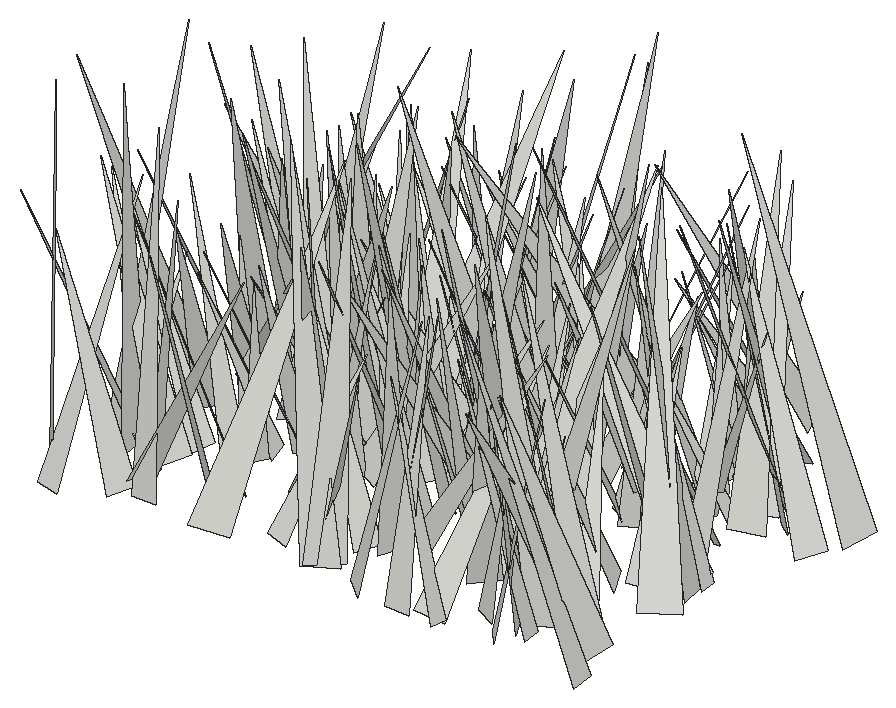
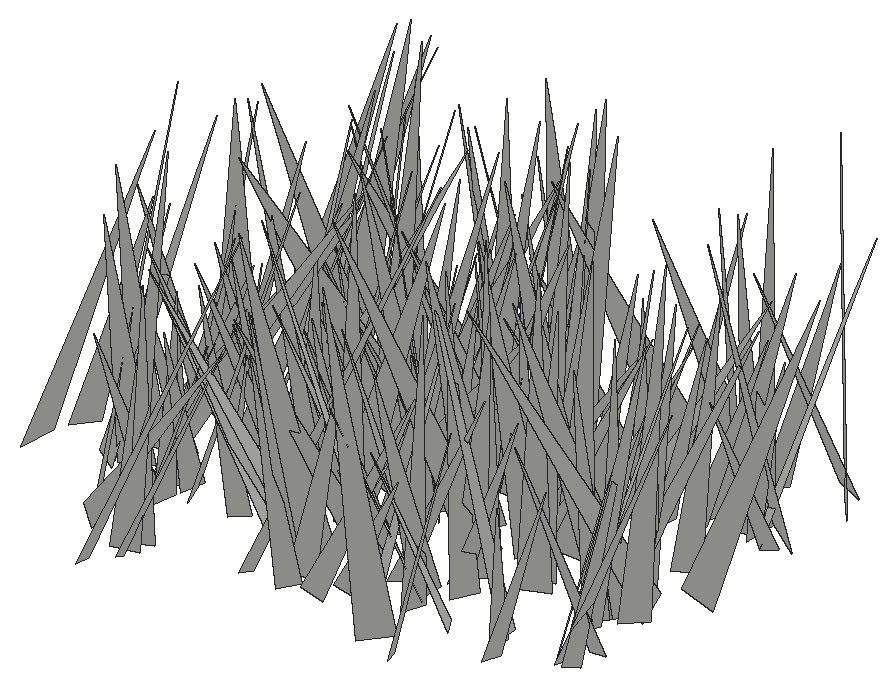
# SketchUp Ruby script. Lengths in inches.
U = 1.inch
M = Sketchup.active_model
def pt(a) = Geom::Point3d.new(a.map { |v| v * U })
def face(e, loops, mat)
  f = e.add_face(loops[0].map { |a| pt(a) })
  loops[1..].each { |l| e.add_face(l.map { |a| pt(a) }).erase! }
  f.material = f.back_material = mat if mat
  f
end
# faces: each face lists its corners as indices into pts; further lists are holes
def faces(e, pts, list, mat = nil) = list.each { |f| face(e, (f[0].is_a?(Array) ? f : [f]).map { |l| l.map { |i| pts[i] } }, mat) }
# xy, xz, yz: faces in a plane at the given z, y or x. An outline is a flat list of corners, or four numbers for a rectangle; further outlines are holes
def ring(l) = l.size == 4 ? [[l[0], l[1]], [l[2], l[1]], [l[2], l[3]], [l[0], l[3]]] : l.each_slice(2).to_a
def flat(e, list, mat, &to3) = list.each { |f| face(e, (f[0].is_a?(Array) ? f : [f]).map { |l| ring(l).map { |u, v| to3.(u, v) } }, mat) }
def xy(e, z, list, mat = nil) = flat(e, list, mat) { |x, y| [x, y, z] }
def xz(e, y, list, mat = nil) = flat(e, list, mat) { |x, z| [x, y, z] }
def yz(e, x, list, mat = nil) = flat(e, list, mat) { |y, z| [x, y, z] }
def lines(e, pts, list) = list.each { |a, b| e.add_line(pt(pts[a]), pt(pts[b])) }
# prism: a flat outline (further loops are holes) pulled along v
def prism(e, loops, v, mat = nil)
  f = face(e, loops, mat); d = Geom::Vector3d.new(v.map { |x| x * U })
  f.pushpull(f.normal.samedirection?(d) ? d.length : -d.length)
end
def box(e, o, s, mat = nil) = prism(e, [[o, [o[0] + s[0], o[1], o[2]], [o[0] + s[0], o[1] + s[1], o[2]], [o[0], o[1] + s[1], o[2]]]], [0, 0, s[2]], mat)
def at(x, y, z, deg = 0) = Geom::Transformation.translation(pt([x, y, z])) * Geom::Transformation.rotation(ORIGIN, Z_AXIS, deg.degrees)
def axes(o, x, y, z) = Geom::Transformation.new([*x, 0, *y, 0, *z, 0, *pt(o).to_a, 1])
def part(name) = M.definitions.add(name)
# library, detail: a bought-in or finely detailed component or shape, given as its bounding box
def library(name, o, s) = part(name).tap { |d| box(d.entities, o, s) }
def detail(e, o, s) = box(e.add_group.entities, o, s)
def put(e, d, t, mat = nil) = e.add_instance(d, t).tap { |i| i.material = mat if mat }
def group(e, t, mat = nil) = e.add_group.tap { |g| g.transformation = t; g.material = mat if mat }.entities
root = M.entities
c1 = part("fur_instance\#9")
p = [[0.8125,0,1.79],[0.67,-0.02,1.48],[0,-0.11,0],[0,0.11,0]]
faces(c1.entities,p,[[0,1,2,3]])
put(root,c1,axes([89.13,415.83,-27.1],[5.01755,-2.86523,2.69296],[-2.1597,-5.65647,-1.99435],[-3.28592,-0.6574,5.42291]))
put(root,c1,axes([90.02,413.82,-27.1],[-7.1325,-1.97369,0.04131],[-1.9512,7.0246,-1.27181],[-0.29997,1.23662,7.29044]))
put(root,c1,axes([67.68,414.45,-27.1],[-4.78062,2.36193,1.12593],[2.54726,4.73726,0.87783],[0.59826,-1.2963,5.25951]))
put(root,c1,axes([64.64,414.03,-27.1],[-5.7343,-4.84539,3.53032],[-5.45543,6.24306,-0.29262],[2.4858,2.5238,7.50162]))
put(root,c1,axes([71.45,415.38,-27.1],[-3.14093,-4.54056,1.19879],[-4.68857,3.11384,-0.49041],[0.26658,1.26749,5.49924]))
put(root,c1,axes([83.08,413.99,-27.1],[-4.76571,-0.2474,0.30777],[-0.30187,4.68534,-0.90794],[0.25457,0.92426,4.68496]))
put(root,c1,axes([86.31,418.15,-27.1],[4.64507,-4.79979,0.2726],[-4.36308,-4.36804,-2.56373],[-2.01887,-1.6035,6.16782]))
put(root,c1,axes([76.08,415.99,-27.1],[5.21952,0.68023,0.61562],[0.83808,-4.98198,-1.60081],[-0.37326,-1.674,5.01433]))
put(root,c1,axes([79.03,414.06,-27.1],[3.65147,4.43575,1.22236],[4.5601,-3.69672,-0.20725],[-0.61278,-1.07778,5.74161]))
put(root,c1,axes([81.28,413.75,-27.1],[0.82489,5.68831,1.342],[5.81529,-0.93413,0.38496],[-0.58339,-1.2684,5.73491]))
put(root,c1,axes([85.58,415.59,-27.1],[3.95748,1.9361,2.48086],[2.44941,-4.39763,-0.47534],[-1.97573,-1.57388,4.37997]))
put(root,c1,axes([84.11,415.45,-27.1],[-0.58036,-3.55618,1.37675],[-3.59236,0.97706,1.00942],[1.27936,1.13031,3.45894]))
put(root,c1,axes([85.32,414.44,-27.1],[3.56693,3.32971,1.1246],[3.34181,-3.70943,0.38354],[-1.08812,-0.47732,4.86445]))
put(root,c1,axes([67.83,415.27,-27.1],[5.28703,-2.12696,0.17156],[-2.11759,-5.17319,1.12251],[0.26309,1.10465,5.58719]))
put(root,c1,axes([79.96,415.2,-27.1],[5.42096,2.25752,1.64956],[2.38588,-5.61122,-0.16143],[-1.45775,-0.7887,5.87002]))
put(root,c1,axes([65.36,412.92,-27.1],[2.05142,5.93925,0.09208],[5.90467,-2.04959,0.65232],[-0.64654,0.12643,6.2496]))
put(root,c1,axes([86.4,415.33,-27.1],[-5.31837,-1.43549,0.4315],[-1.49067,5.23198,-0.96754],[0.15722,1.04767,5.42306]))
put(root,c1,axes([65.6,418.01,-27.1],[-4.61159,-4.4726,0.38091],[-4.39573,4.61032,0.9157],[0.90928,-0.396,6.35865]))
put(root,c1,axes([77.02,414.81,-27.1],[-5.99811,4.4385,2.51735],[4.45899,6.44808,-0.74453],[2.48087,-0.8583,7.4245]))
put(root,c1,axes([77.01,414.55,-27.1],[-1.50956,7.97784,1.83345],[8.07703,1.14872,1.65178],[-1.3301,-2.07864,7.94961]))
put(root,c1,axes([82.47,417.49,-27.1],[4.37125,-4.19897,0.80164],[-4.19734,-4.43318,-0.33332],[-0.81017,0.31203,6.05212]))
put(root,c1,axes([78.4,417.3,-27.1],[5.51508,-3.1001,1.56666],[-3.03836,-5.73026,-0.64316],[-1.68328,0.18611,6.29389]))
put(root,c1,axes([68.75,414.43,-27.1],[1.63726,6.8228,1.57078],[6.72877,-1.9791,1.58281],[-1.9343,-1.10957,6.83563]))
put(root,c1,axes([74.47,415.16,-27.1],[0.4921,4.23207,0.57816],[4.10963,-0.31046,-1.22532],[1.16432,-0.69285,4.08059]))
put(root,c1,axes([82.51,414.16,-27.1],[-2.22642,5.28944,0.76409],[4.89566,2.35054,-2.00661],[2.14349,0.12554,5.37668]))
put(root,c1,axes([67.1,417.14,-27.1],[3.49606,4.56093,2.47636],[5.16488,-3.35013,-1.12142],[-0.50841,-2.67048,5.63622]))
put(root,c1,axes([86.95,417.37,-27.1],[-5.18557,-4.32883,1.54546],[-4.49087,5.26797,-0.31293],[0.97941,1.23577,6.74766]))
put(root,c1,axes([86.36,416.29,-27.1],[-0.9931,7.68396,2.84346],[8.04191,0.36629,1.81887],[-1.56723,-2.98953,7.53135]))
put(root,c1,axes([77.51,416.75,-27.1],[-4.02277,2.62654,1.01722],[2.78428,3.97624,0.74391],[0.42575,-1.18612,4.74637]))
put(root,c1,axes([65.93,417.47,-27.1],[7.3985,0.06507,3.2704],[0.28828,-8.06925,-0.49163],[-3.25831,-0.56619,7.38244]))
put(root,c1,axes([72.08,414.11,-27.1],[-4.61251,5.93847,1.25396],[5.3205,4.71401,-2.75381],[2.92064,0.79104,6.99694]))
put(root,c1,axes([72.86,420.16,-27.1],[5.93446,-4.51627,0.11992],[-4.41947,-5.84426,-1.3935],[-0.93776,-1.03771,7.32616]))
put(root,c1,axes([71.45,417.04,-27.1],[-4.82792,-3.85999,0.34861],[-3.62589,4.30173,-2.58417],[-1.36894,2.21934,5.6152]))
put(root,c1,axes([67.8,417.46,-27.1],[-5.5849,2.54638,0.93821],[2.66389,5.55377,0.78405],[0.51763,-1.10771,6.08773]))
put(root,c1,axes([78.87,418.1875,-27.1],[4.45492,4.83666,0.95124],[4.56601,-3.56591,-3.25273],[1.85733,-2.83468,5.71483]))
put(root,c1,axes([87.88,416.87,-27.1],[-6.93734,1.12272,0.61983],[1.08478,6.95591,-0.45824],[0.68406,0.3553,7.01265]))
put(root,c1,axes([84.2,417.5625,-27.1],[-6.46812,-3.13785,1.21731],[-3.3431,6.29489,-1.53709],[0.38946,1.92167,7.02282]))
put(root,c1,axes([76.34,421.15,-27.1],[-2.99336,-6.46525,0.18966],[-6.30073,2.9619,1.52434],[1.46161,-0.47255,6.9596]))
put(root,c1,axes([74.34,418.125,-27.1],[-5.53367,-3.1899,2.46645],[-3.58117,5.81278,-0.51687],[1.85312,1.70777,6.3663]))
put(root,c1,axes([80.82,418.96,-27.1],[-3.26871,-2.2439,0.63682],[-2.29753,3.28654,-0.21245],[0.40248,0.53729,3.95909]))
put(root,c1,axes([74.2,418.54,-27.1],[-1.49797,-4.88201,2.75569],[-5.27998,2.18724,1.00478],[1.88406,2.24805,5.00683]))
put(root,c1,axes([70.18,419.33,-27.1],[3.44775,-2.42349,1.09947],[-2.43313,-3.5995,-0.30427],[-1.07797,0.37336,4.2033]))
put(root,c1,axes([80.49,419.33,-27.1],[-1.33118,-5.02308,1.66852],[-5.29255,1.28443,-0.35575],[0.06525,1.70478,5.18429]))
put(root,c1,axes([80.43,421.6,-27.1],[7.22069,-3.00234,1.05262],[-2.62839,-7.10035,-2.22196],[-1.79266,-1.6827,7.49769]))
put(root,c1,axes([86.3,420.58,-27.1],[-5.06216,-2.56794,0.53616],[-2.44101,5.03776,1.08155],[0.96086,-0.73072,5.57226]))
put(root,c1,axes([83.34,419.48,-27.1],[3.34183,1.38887,0.77255],[1.56239,-3.2005,-1.00466],[-0.29109,-1.23347,3.4767]))
put(root,c1,axes([67.99,418.83,-27.1],[-4.93751,1.50851,0.32737],[1.53378,4.91815,0.47027],[0.1741,-0.54591,5.14135]))
put(root,c1,axes([66.37,417.86,-27.1],[-3.43494,4.07646,0.13435],[4.04677,3.38429,0.77755],[-0.50915,-0.60283,5.27368]))
put(root,c1,axes([70.38,420.34,-27.1],[-4.26767,-0.91045,0.71231],[-0.70932,4.21373,1.13607],[0.91278,-0.98229,4.21323]))
put(root,c1,axes([79.55,421.67,-27.1],[1.60402,-6.13136,0.73735],[-5.58582,-1.76536,-2.52831],[-2.63361,0.00991,5.81155]))
put(root,c1,axes([78.98,418.61,-27.1],[-7.05105,-1.29004,0.36767],[-1.33665,6.92247,-1.34515],[0.11284,1.38992,7.04075]))
put(root,c1,axes([64.91,418.23,-27.1],[-0.81178,3.59213,0.55552],[3.51446,0.92094,-0.81938],[0.92765,-0.34562,3.5904]))
put(root,c1,axes([84.94,419.75,-27.1],[-4.9499,-5.12629,0.49866],[-4.98162,4.58947,-2.26921],[-1.30806,1.92014,6.75508]))
put(root,c1,axes([84.68,417.39,-27.1],[6.67924,-1.26552,2.75336],[-2.18749,-6.62541,2.26131],[-2.097,2.88046,6.41095]))
put(root,c1,axes([71.25,420.98,-27.1],[1.69834,-4.62751,0.65795],[-4.61755,-1.76962,-0.52709],[-0.72459,0.43091,4.90106]))
put(root,c1,axes([66.21,421.51,-27.1],[3.84252,-3.67557,0.42443],[-3.56655,-3.84235,-0.9854],[-0.98471,-0.42605,5.2253]))
put(root,c1,axes([75.875,420.37,-27.1],[-6.16765,-3.82155,1.90605],[-3.98751,6.35208,-0.16723],[1.52874,1.15063,7.2537]))
put(root,c1,axes([81.23,419.77,-27.1],[-3.53133,-2.30027,1.49102],[-2.55807,3.63918,-0.44418],[0.98523,1.20406,4.19097]))
put(root,c1,axes([71.56,420.58,-27.1],[-3.04212,-3.44962,0.11938],[-3.35963,2.92271,-1.15727],[-0.79185,0.85236,4.45141]))
put(root,c1,axes([65.06,417.26,-27.1],[3.59561,7.30217,1.1805],[7.09033,-3.77639,1.76345],[-2.10771,-0.24675,7.94609]))
put(root,c1,axes([72.86,420.31,-27.1],[1.59006,-7.38899,3.46765],[-7.94346,-2.21328,-1.07372],[-1.87702,3.10714,7.48148]))
put(root,c1,axes([69.16,419.22,-27.1],[-5.26641,1.25593,0.32091],[1.22212,5.2582,-0.5227],[0.43216,0.43524,5.3888]))
put(root,c1,axes([86.23,418.76,-27.1],[-2.52047,3.62206,0.22803],[3.61381,2.53037,-0.24846],[0.33426,-0.04477,4.40572]))
put(root,c1,axes([72.46,418.55,-27.1],[4.05537,2.07279,0.17475],[1.9711,-3.95155,1.12829],[-0.66463,0.92835,4.41242]))
put(root,c1,axes([73.86,420.27,-27.1],[-6.94561,0.7265,2.56424],[0.79665,7.39636,0.06233],[2.54332,-0.33278,6.98322]))
put(root,c1,axes([82.72,418.65,-27.1],[1.79845,4.31058,0.12569],[4.2592,-1.79684,0.67963],[-0.67534,0.14702,4.621]))
put(root,c1,axes([78.66,422.29,-27.1],[-0.3519,-5.66898,0.64957],[-5.59847,0.21723,-1.13712],[-1.1029,0.70611,5.5649]))
put(root,c1,axes([76.5,420.01,-27.1],[2.39277,4.07076,1.54907],[4.21231,-2.6123,0.35825],[-1.10775,-1.14055,4.7083]))
put(root,c1,axes([74.09,421.6,-27.1],[-1.49578,-4.28811,0.26565],[-3.87905,1.22698,-2.03551],[-1.84701,0.89578,4.0598]))
put(root,c1,axes([82.9,424.91,-27.1],[-3.72735,-5.65721,0.3773],[-4.71825,3.34531,3.54775],[3.14396,-1.68653,5.77153]))
put(root,c1,axes([78.07,420.84,-27.1],[-2.85535,-4.62994,1.75531],[-4.89429,2.33192,-1.81068],[-0.75056,2.40755,5.12941]))
put(root,c1,axes([66.88,423.35,-27.1],[4.17409,-3.35782,0.27535],[-3.2273,-4.11088,-1.20788],[-0.96712,-0.77425,5.2191]))
put(root,c1,axes([75.68,422.91,-27.1],[0.67121,-5.58126,0.90748],[-5.6399,-0.72653,-0.2969],[-0.40679,0.86382,5.61363]))
put(root,c1,axes([74.67,423.49,-27.1],[-1.5232,-7.73744,1.34983],[-7.81047,1.63722,0.57115],[0.82858,1.20901,7.86523]))
put(root,c1,axes([67.85,422.62,-27.1],[-3.27123,-4.88451,0.3113],[-4.82797,3.15879,-1.17003],[-0.80376,0.90546,5.76111]))
put(root,c1,axes([70.71,422.39,-27.1],[5.42547,-4.53511,0.52895],[-4.56014,-5.3411,0.98008],[0.2284,1.09004,7.00303]))
put(root,c1,axes([81.42,423.81,-27.1],[-5.10979,-2.8974,1.28802],[-2.4355,5.15064,1.92434],[2.03034,-1.11347,5.54994]))
put(root,c1,axes([86.8,422.77,-27.1],[-2.84226,-5.05917,1.08036],[-5.16298,2.85167,-0.22901],[0.32566,1.05526,5.79838]))
put(root,c1,axes([81.97,420.52,-27.1],[0.88242,4.55252,0.64978],[4.54635,-0.76413,-0.82042],[0.6916,-0.78549,4.5641]))
put(root,c1,axes([73.89,421,-27.1],[1.55014,5.60518,1.20615],[5.3228,-0.94254,-2.46072],[2.13086,-1.72318,5.26933]))
put(root,c1,axes([76.1875,422.26,-27.1],[-3.70212,4.89762,1.86065],[5.19102,3.12087,2.11373],[-0.70854,-2.72541,5.76407]))
put(root,c1,axes([64.6,422.91,-27.1],[-0.79345,-6.87819,1.77521],[-6.83318,0.25089,-2.08208],[-1.94125,1.92821,6.60333]))
put(root,c1,axes([89.12,421.49,-27.1],[-6.73527,-1.87686,1.53677],[-2.12146,6.75676,-1.04577],[1.17629,1.43931,6.91323]))
put(root,c1,axes([89.02,419.68,-27.1],[-3.36629,7.35026,0.38103],[7.33966,3.3212,0.77612],[-0.54849,-0.66835,8.0471]))
put(root,c1,axes([67.26,422.54,-27.1],[1.04159,-3.44564,1.2731],[-3.64709,-1.12789,-0.06873],[-0.4381,1.19732,3.59897]))
put(root,c1,axes([75.13,421.11,-27.1],[-0.50295,4.78104,0.71911],[4.81704,0.43358,0.48636],[-0.41423,-0.76294,4.78276]))
put(root,c1,axes([89.18,422.36,-27.1],[-3.86057,-0.50737,0.50019],[-0.53854,3.88252,-0.21837],[0.46646,0.28336,3.88764]))
put(root,c1,axes([82.76,418.35,-27.1],[-6.00676,5.62271,0.83771],[4.81686,5.68135,-3.59416],[3.01902,2.12255,7.40122]))
put(root,c1,axes([87.07,420.76,-27.1],[0.03105,4.61747,0.04613],[4.59439,-0.03553,0.46309],[-0.46341,-0.04278,4.59429]))
put(root,c1,axes([77.5,424.12,-27.1],[3.26712,2.26093,2.86418],[3.20778,-3.61207,-0.80776],[-1.73938,-2.41465,3.89016]))
put(root,c1,axes([88.39,422.87,-27.1],[-2.47066,2.78913,0.64805],[2.82871,2.24449,1.12431],[-0.44456,-1.21919,3.55237]))
put(root,c1,axes([76.47,422.72,-27.1],[-0.19493,4.51759,1.73565],[4.75586,-0.14282,0.90585],[-0.89608,-1.74071,4.43013]))
put(root,c1,axes([78.51,423.77,-27.1],[-2.5232,4.5633,1.53247],[4.25008,1.29942,3.12842],[-2.26029,-2.65076,4.17172]))
put(root,c1,axes([76.4,422.45,-27.1],[1.55212,3.88569,0.28277],[3.69063,-1.36892,-1.44671],[1.24813,-0.78428,3.92616]))
put(root,c1,axes([77.59,422.46,-27.1],[6.54484,-1.1484,2.12677],[-1.53141,-6.71985,1.08414],[-1.86996,1.48383,6.55579]))
put(root,c1,axes([88.48,422.34,-27.1],[-3.77529,6.85051,0.02559],[5.94676,3.26269,3.89536],[-3.40091,-1.89957,6.78296]))
put(root,c1,axes([72.57,422.9,-27.1],[-0.09344,5.23116,1.72248],[5.50098,0.0052,0.28262],[-0.26677,-1.725,5.22436]))
put(root,c1,axes([76.12,423.83,-27.1],[6.04593,4.4435,2.18806],[4.86244,-5.98205,-1.28733],[-0.94282,-2.35709,7.39194]))
put(root,c1,axes([71.57,423.94,-27.1],[-3.32714,-4.87132,0.7615],[-4.7527,2.92423,-2.05917],[-1.31203,1.7603,5.52806]))
put(root,c1,axes([84.7,424.87,-27.1],[-1.00098,-5.50903,0.83943],[-5.47181,0.81017,-1.20786],[-1.05515,1.02481,5.46739]))
put(root,c1,axes([65.36,425.7,-27.1],[6.33398,-2.31725,1.64534],[-1.9481,-6.46653,-1.60778],[-2.06922,-1.00519,6.55011]))
put(root,c1,axes([66.53,426.39,-27.1],[6.05103,1.03829,2.78411],[2.19851,-5.8136,-2.61017],[-1.99898,-3.2509,5.55698]))
put(root,c1,axes([80.48,422.68,-27.1],[0.12612,4.07155,0.3622],[4.08216,-0.1442,0.19951],[-0.2114,-0.35539,4.06861]))
put(root,c1,axes([82.58,423.27,-27.1],[-4.08375,3.22336,1.0157],[3.24667,4.18417,-0.22495],[0.93853,-0.4488,5.19774]))
put(root,c1,axes([70.18,423.24,-27.1],[-1.69454,7.12423,1.83382],[7.32335,1.45532,1.11334],[-0.69716,-2.02889,7.23786]))
put(root,c1,axes([76.58,426.27,-27.1],[-7.9399,0.37328,2.34081],[0.92834,8.01881,1.87016],[2.18103,-2.05426,7.72553]))
put(root,c1,axes([71.34,424.11,-27.1],[-3.27295,5.40819,2.7555],[5.57889,3.91368,-1.05481],[2.39109,-1.7286,6.23283]))
put(root,c1,axes([81.21,424.77,-27.1],[-2.12698,-6.60371,3.80122],[-7.1046,3.14508,1.48842],[2.75369,3.0136,6.77625]))
put(root,c1,axes([66.2,426.08,-27.1],[5.00192,-1.81934,1.03799],[-1.65,-5.07776,-0.94895],[-1.29032,-0.55947,5.23724]))
put(root,c1,axes([76.47,423.64,-27.1],[-1.50833,4.20798,0.27956],[4.21722,1.50618,0.08227],[0.01672,-0.29093,4.46939]))
put(root,c1,axes([70.14,425.34,-27.1],[1.65081,-5.08845,2.41171],[-5.51574,-1.96719,-0.37505],[-1.13372,2.16141,5.33637]))
put(root,c1,axes([87.43,425.06,-27.1],[-5.76145,-5.93812,0.42997],[-5.44241,5.01036,-3.73055],[-2.41379,2.87671,7.38502]))
put(root,c1,axes([67.625,425.51,-27.1],[-5.88104,-3.53705,0.94417],[-3.64814,5.81133,-0.9531],[0.30541,1.30636,6.79625]))
put(root,c1,axes([78.9375,425.68,-27.1],[-0.03383,-6.90938,2.82252],[-7.12958,-0.80509,-2.05628],[-2.20801,2.70547,6.5964]))
put(root,c1,axes([69.74,426.18,-27.1],[2.04038,-5.82637,1.87095],[-6.1057,-2.07021,0.21174],[-0.4092,1.83789,6.16967]))
put(root,c1,axes([87.95,422.89,-27.1],[1.53889,6.65129,0.3221],[6.53467,-1.57198,1.24039],[-1.28121,-0.02868,6.71336]))
put(root,c1,axes([83.02,424.69,-27.1],[1.48501,3.27806,0.44782],[3.28348,-1.52047,0.24164],[-0.40618,-0.30651,3.59062]))
put(root,c1,axes([69.33,422.63,-27.1],[-6.96616,2.88196,1.8212],[2.05018,6.85162,-3.00033],[2.72382,2.21349,6.91601]))
put(root,c1,axes([66.6,426.34,-27.1],[2.66304,-4.00114,1.09323],[-4.14622,-2.60379,0.57024],[-0.11461,1.22768,4.77239]))
put(root,c1,axes([71.75,426.38,-27.1],[-0.58668,-6.43534,2.37936],[-6.81319,0.82822,0.56013],[0.80964,2.30643,6.43771]))
put(root,c1,axes([67.8,425.375,-27.1],[-4.98087,1.16288,0.32288],[1.15979,4.99131,-0.08543],[0.33384,0.00996,5.1141]))
put(root,c1,axes([78.16,426.57,-27.1],[0.12589,-6.48138,2.39431],[-6.90548,-0.03647,0.26437],[0.23531,2.39734,6.47721]))
put(root,c1,axes([86.71,426.96,-27.1],[-3.57731,-0.93265,0.01118],[-0.92223,3.54345,0.51048],[0.1395,-0.49118,3.66148]))
put(root,c1,axes([88.41,428.24,-27.1],[-4.17901,-5.88434,0.7845],[-5.89024,4.22956,0.34775],[0.73891,0.43633,7.20893]))
put(root,c1,axes([74.07,423.74,-27.1],[-5.45003,5.37343,0.92209],[5.18096,5.51046,-1.48977],[1.69756,0.43353,7.50714]))
put(root,c1,axes([85.92,426.39,-27.1],[4.29201,-0.29938,0.77765],[-0.39482,-4.32378,0.51456],[-0.73381,0.57535,4.27156]))
put(root,c1,axes([83.32,427.26,-27.1],[-4.36965,-1.59831,1.51111],[-1.58231,4.61869,0.30967],[1.52785,0.21216,4.64247]))
put(root,c1,axes([80.67,426.51,-27.1],[0.36945,4.73641,1.83647],[4.53767,0.52011,-2.25427],[2.28381,-1.79961,4.18191]))
put(root,c1,axes([66.42,427.25,-27.1],[-6.02827,1.48886,1.73676],[1.72693,6.17226,0.7029],[1.50026,-1.12234,6.1695]))
put(root,c1,axes([72.23,426.88,-27.1],[-4.31803,3.62073,2.04082],[3.93255,4.51165,0.31626],[1.34522,-1.56695,5.62628]))
put(root,c1,axes([71.5,428.05,-27.1],[5.97247,-1.71505,1.0533],[-1.60325,-6.04797,-0.7569],[-1.21673,-0.44932,6.16757]))
put(root,c1,axes([65.51,424.48,-27.1],[7.33228,1.89466,0.16833],[1.78282,-7.07911,2.02191],[-0.66303,1.91751,7.29821]))
put(root,c1,axes([90.7,426.59,-27.1],[-5.38349,2.8617,0.60302],[2.91403,5.35589,0.59819],[0.24775,-0.81245,6.06741]))
put(root,c1,axes([77.83,427.02,-27.1],[-3.1989,2.68909,0.37978],[2.66785,3.00183,1.21655],[-0.50792,-1.16886,3.99802]))
put(root,c1,axes([87.21,430.11,-27.1],[-6.01376,-4.74049,2.00405],[-3.98095,6.23797,2.80955],[3.26197,-1.12665,7.12348]))
put(root,c1,axes([84.18,428.32,-27.1],[-6.24569,-2.79636,0.92417],[-2.76847,6.31368,0.39421],[1.00464,0.01396,6.83176]))
put(root,c1,axes([84.02,424.07,-27.1],[2.20032,6.76237,0.49836],[6.15454,-2.21163,2.83722],[-2.84601,0.44546,6.52083]))
put(root,c1,axes([73.3,424.84,-27.1],[-0.97355,8.05143,1.14446],[7.84551,1.23329,-2.00251],[2.14086,-0.85824,7.85896]))
put(root,c1,axes([72.33,427.375,-27.1],[-3.83694,1.86592,0.39498],[1.90547,3.78872,0.61201],[0.08273,-0.72368,4.22246]))
put(root,c1,axes([78.17,425.41,-27.1],[4.5765,3.32185,0.66717],[3.07667,-4.544,1.52],[-1.41913,0.86116,5.4469]))
put(root,c1,axes([79,431.66,-27.1],[-7.67561,-3.02253,0.64542],[-2.50236,7.09168,3.4516],[1.81396,-3.00659,7.49247]))
put(root,c1,axes([88.69,427.51,-27.1],[2.96491,4.33641,3.25393],[4.46173,-4.05854,1.34327],[-3.07985,-1.70497,5.07846]))
put(root,c1,axes([75.94,427.99,-27.1],[3.19259,1.80159,0.09548],[1.75198,-3.04965,-1.03811],[0.43061,-0.9494,3.51578]))
put(root,c1,axes([65.07,429.78,-27.1],[-4.32761,-0.50237,2.11035],[0.41917,4.42689,1.9134],[2.12844,-1.89326,3.91401]))
put(root,c1,axes([65.59,429.66,-27.1],[-5.22696,-1.19875,0.73288],[-0.94186,5.08442,1.59898],[1.04259,-1.41663,5.11873]))
put(root,c1,axes([85.04,428.0625,-27.1],[-2.3678,2.48019,1.72309],[2.76192,2.66404,-0.03926],[1.22155,-1.2159,3.42875]))
put(root,c1,axes([81.79,428.54,-27.1],[1.56073,-4.1385,0.9971],[-4.17951,-1.28812,1.1957],[0.80812,1.33073,4.25833]))
put(root,c1,axes([75.71,427.31,-27.1],[4.89085,0.64493,0.58721],[0.56841,-4.89366,0.64042],[-0.66156,0.56328,4.89144]))
put(root,c1,axes([77.01,427.64,-27.1],[-2.42701,4.03219,1.90827],[4.11447,2.86278,-0.81615],[1.72373,-1.15601,4.63496]))
put(root,c1,axes([65.98,429.43,-27.1],[-3.08221,-2.2445,0.63722],[-2.14243,3.14072,0.69983],[0.92405,-0.20483,3.74807]))
put(root,c1,axes([87.73,426.46,-27.1],[-1.40207,7.22786,1.13046],[7.31414,1.36087,0.37039],[-0.15287,-1.17973,7.35327]))
put(root,c1,axes([74.11,428.68,-27.1],[-4.51711,1.79985,0.33219],[1.82954,4.41557,0.95372],[-0.05124,-1.00862,4.76803]))
put(root,c1,axes([74.78,426.85,-27.1],[4.77639,3.07128,1.21309],[2.81816,-4.90311,1.31748],[-1.72115,0.49496,5.52367]))
put(root,c1,axes([68.45,429.32,-27.1],[6.75177,1.95337,0.7466],[2.07523,-6.56983,-1.57805],[-0.25785,-1.72661,6.84922]))
put(root,c1,axes([91.35,428.625,-27.1],[-8.2127,0.65784,0.53458],[0.66874,8.22786,0.14871],[0.52088,-0.19122,8.23766]))
put(root,c1,axes([85.98,428.65,-27.1],[-4.15206,-1.52587,0.16301],[-1.50616,3.96212,-1.27574],[-0.29385,1.25209,4.2356]))
put(root,c1,axes([72.42,429.96,-27.1],[5.48977,-0.87036,1.92832],[-0.64898,-5.79667,-0.76876],[-2.01365,-0.50463,5.50492]))
put(root,c1,axes([80.62,428.27,-27.1],[4.47916,2.33614,0.04477],[2.33654,-4.47877,-0.05982],[-0.01203,-0.07375,5.05142]))
put(root,c1,axes([72.76,432.33,-27.1],[-3.43989,-5.36661,0.1848],[-4.97328,3.26677,2.29397],[2.02515,-1.09328,5.94736]))
put(root,c1,axes([80.82,427.99,-27.1],[5.67742,2.27779,0.25934],[2.25803,-5.67581,0.41845],[-0.39608,0.29237,6.10297]))
put(root,c1,axes([64.92,428.41,-27.1],[1.35315,4.35582,0.79538],[4.34518,-1.14634,-1.11449],[0.85157,-1.07217,4.42291]))
put(root,c1,axes([84.51,427.95,-27.1],[-3.56654,2.39752,0.7344],[2.22273,3.6139,-1.00345],[1.16058,0.44646,4.17868]))
put(root,c1,axes([87.25,427.84,-27.1],[-2.49742,5.95651,1.04282],[6.02179,2.55284,-0.16018],[0.55273,-0.89868,6.45689]))
put(root,c1,axes([84.79,429.3,-27.1],[-4.53937,1.16522,1.40638],[1.15678,4.75002,-0.2018],[1.41333,-0.14527,4.6822]))
put(root,c1,axes([75.87,428.02,-27.1],[6.07013,4.91373,1.22638],[4.90353,-6.18107,0.495],[-1.26656,-0.38061,7.79399]))
put(root,c1,axes([79.71,427.85,-27.1],[5.6659,3.07924,0.02777],[3.03508,-5.59401,1.03936],[-0.52039,0.90013,6.36426]))
put(root,c1,axes([75.3,428.51,-27.1],[5.97099,-0.01983,0.33196],[-0.11666,-5.7151,1.75709],[-0.31141,1.76085,5.70664]))
put(root,c1,axes([83.57,433.15,-27.1],[-0.94018,-7.50089,0.47804],[-7.29693,1.02641,1.75419],[1.80188,0.24278,7.35324]))
put(root,c1,axes([76.66,430.65,-27.1],[-2.71564,-2.49022,0.0198],[-2.39499,2.6036,-1.03032],[-0.68234,0.77224,3.53756]))
put(root,c1,axes([72.93,428.98,-27.1],[2.99625,3.60782,0.19235],[3.59342,-3.00177,0.328],[-0.37513,0.06212,4.67828]))
put(root,c1,axes([76.03,431.48,-27.1],[0.12283,-4.44104,1.09952],[-4.1986,-0.54638,-1.73783],[-1.81756,0.96203,4.08875]))
put(root,c1,axes([72.66,428.87,-27.1],[4.91626,-1.03874,2.91243],[-2.03601,-5.20453,1.58061],[-2.3272,2.35896,4.76972]))
put(root,c1,axes([83.875,432.13,-27.1],[-3.49973,-1.74713,0.54329],[-1.50598,3.41664,1.28623],[1.03907,-0.93268,3.69408]))
put(root,c1,axes([85.03,429.63,-27.1],[3.51726,-1.23078,1.44078],[-1.67757,-3.4351,1.16087],[-0.88116,1.62697,3.54095]))
put(root,c1,axes([77.2,430.62,-27.1],[1.69917,-3.99461,2.49122],[-4.30676,-2.38859,-0.89256],[-1.90128,1.84064,4.24822]))
put(root,c1,axes([77.07,431.52,-27.1],[3.70766,-2.56946,0.56874],[-2.62102,-3.69364,0.39947],[-0.23628,0.65362,4.49325]))
put(root,c1,axes([67.79,431.13,-27.1],[-4.13289,0.76106,0.51137],[0.79822,4.14817,0.27763],[0.45116,-0.36746,4.1932]))
put(root,c1,axes([70.53,430.19,-27.1],[3.48298,2.03603,0.22687],[2.02285,-3.48877,0.25421],[-0.32396,0.10555,4.02641]))
put(root,c1,axes([77.51,429.35,-27.1],[-6.57541,3.25527,2.97746],[2.73361,7.20101,-1.83599],[3.46258,0.49673,7.10365]))
put(root,c1,axes([68.23,430.17,-27.1],[-3.61922,1.27993,0.57976],[1.16278,3.62754,-0.74965],[0.78884,0.52519,3.76496]))
put(root,c1,axes([83.35,432.47,-27.1],[1.74282,-4.6233,0.69197],[-4.67126,-1.6936,0.44965],[0.18179,0.80496,4.92038]))
put(root,c1,axes([75.23,430.55,-27.1],[-1.27036,4.00789,0.19304],[3.62684,1.0603,1.85365],[-1.71652,-0.72583,3.77372]))
put(root,c1,axes([86.24,432.01,-27.1],[-2.89235,-4.23355,0.19447],[-3.82387,2.50545,-2.32964],[-1.82723,1.45817,4.56743]))
put(root,c1,axes([83.37,433.7,-27.1],[-4.08154,-1.42978,0.42723],[-1.12455,3.76494,1.85644],[0.98091,-1.633,3.906]))
put(root,c1,axes([72.06,432.6,-27.1],[4.17452,-5.37379,1.20818],[-5.50555,-4.02647,1.11376],[0.16212,1.6352,6.71296]))
put(root,c1,axes([84.24,434.83,-27.1],[-6.53247,-2.60599,0.49941],[-2.30056,6.22381,2.3844],[1.32211,-2.04617,6.61657]))
put(root,c1,axes([78.19,429.89,-27.1],[2.36714,6.37429,1.14743],[6.22522,-2.57637,1.46983],[-1.78738,-0.5313,6.63886]))
put(root,c1,axes([70.78,433.35,-27.1],[-3.9819,-2.09854,0.99873],[-1.89028,4.07705,1.03024],[1.35209,-0.4803,4.38155]))
